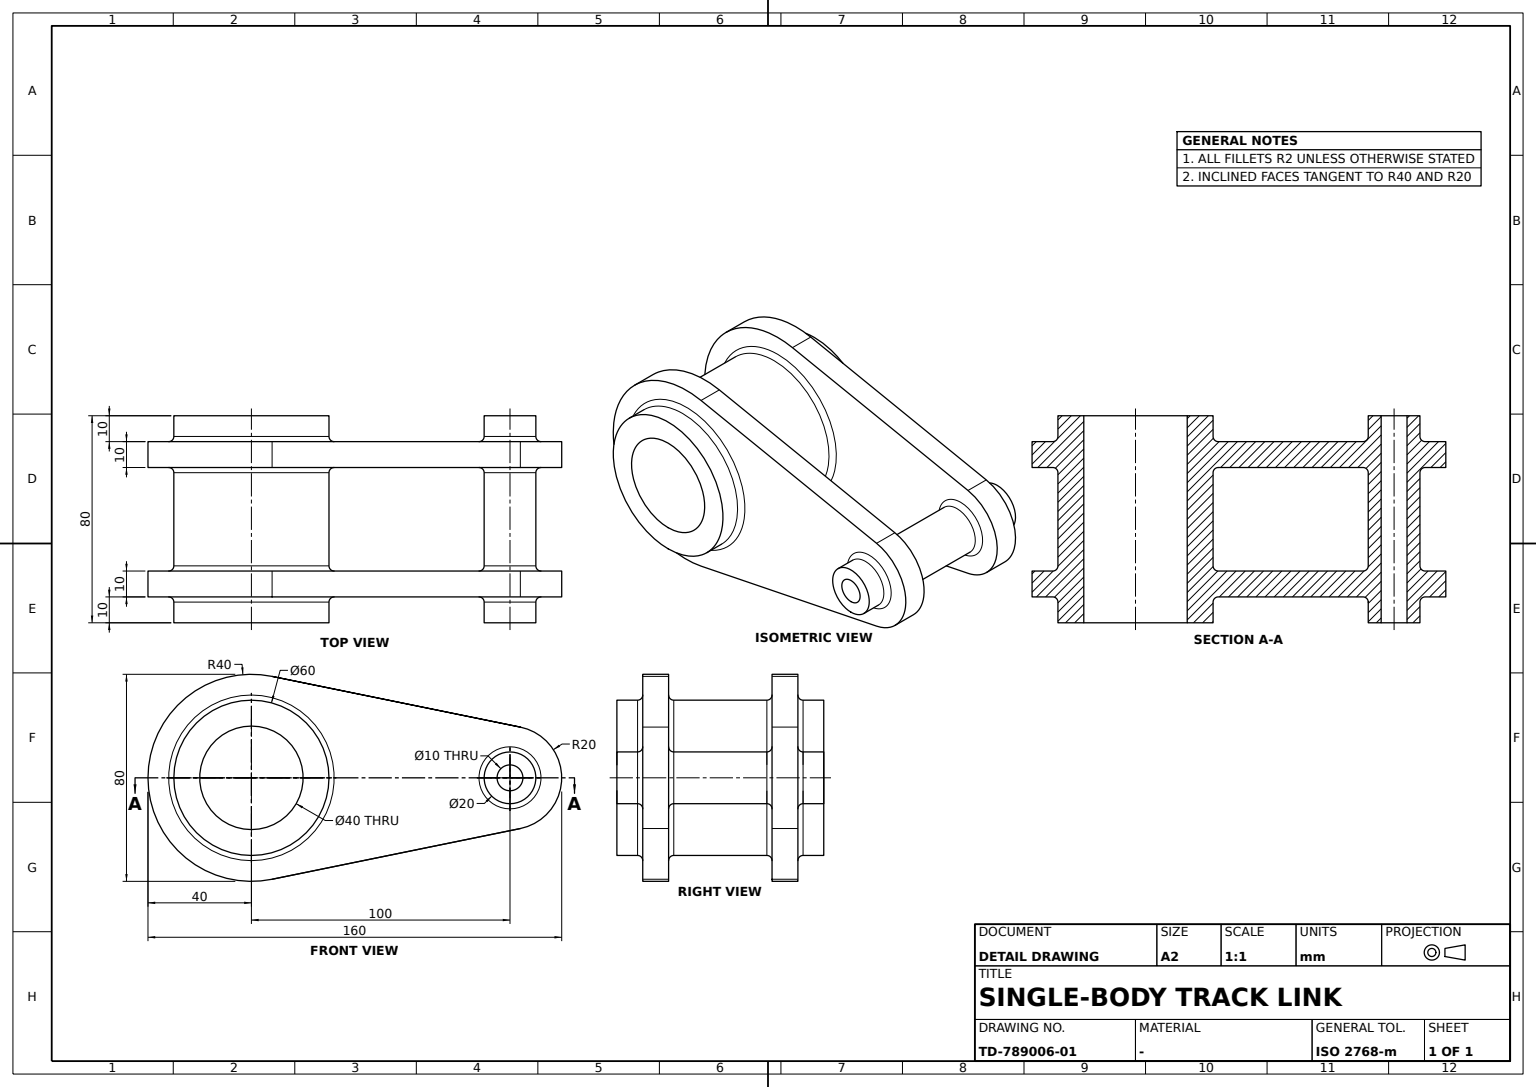
ISO-10303-21;
HEADER;
FILE_DESCRIPTION((''),'2;1');
FILE_NAME('','',(''),(''),'','','');
FILE_SCHEMA(('AUTOMOTIVE_DESIGN'));
ENDSEC;
DATA;
#1=APPLICATION_CONTEXT('');
#2=PRODUCT_CONTEXT('',#1,'mechanical');
#3=PRODUCT('','','',(#2));
#4=PRODUCT_DEFINITION_FORMATION('','',#3);
#5=PRODUCT_DEFINITION_CONTEXT('',#1,'design');
#6=PRODUCT_DEFINITION('','',#4,#5);
#7=PRODUCT_DEFINITION_SHAPE('','',#6);
#8=(LENGTH_UNIT()NAMED_UNIT(*)SI_UNIT(.MILLI.,.METRE.));
#9=(NAMED_UNIT(*)PLANE_ANGLE_UNIT()SI_UNIT($,.RADIAN.));
#10=(NAMED_UNIT(*)SI_UNIT($,.STERADIAN.)SOLID_ANGLE_UNIT());
#11=UNCERTAINTY_MEASURE_WITH_UNIT(LENGTH_MEASURE(0.005),#8,'distance_accuracy_value','');
#12=(GEOMETRIC_REPRESENTATION_CONTEXT(3)GLOBAL_UNCERTAINTY_ASSIGNED_CONTEXT((#11))GLOBAL_UNIT_ASSIGNED_CONTEXT((#8,#9,#10))REPRESENTATION_CONTEXT('',''));
#13=CARTESIAN_POINT('',(0.,103.999996,19.595919));
#14=VERTEX_POINT('',#13);
#15=CARTESIAN_POINT('',(10.,104.,19.595918));
#16=VERTEX_POINT('',#15);
#17=CARTESIAN_POINT('',(-45.,104.,19.595918));
#18=DIRECTION('',(-1.,0.,0.));
#19=VECTOR('',#18,1000.);
#20=LINE('',#17,#19);
#21=EDGE_CURVE('',#14,#16,#20,.F.);
#22=ORIENTED_EDGE('',*,*,#21,.F.);
#23=CARTESIAN_POINT('',(0.,8.,39.191836));
#24=VERTEX_POINT('',#23);
#25=DIRECTION('',(0.,0.979795897,-0.2));
#26=VECTOR('',#25,1000.);
#27=LINE('',#23,#26);
#28=EDGE_CURVE('',#24,#14,#27,.T.);
#29=ORIENTED_EDGE('',*,*,#28,.F.);
#30=CARTESIAN_POINT('',(10.,8.000004,39.191835));
#31=VERTEX_POINT('',#30);
#32=CARTESIAN_POINT('',(-45.,8.,39.191836));
#33=LINE('',#32,#19);
#34=EDGE_CURVE('',#24,#31,#33,.F.);
#35=ORIENTED_EDGE('',*,*,#34,.T.);
#36=CARTESIAN_POINT('',(10.,8.,39.191836));
#37=LINE('',#36,#26);
#38=EDGE_CURVE('',#31,#16,#37,.T.);
#39=ORIENTED_EDGE('',*,*,#38,.T.);
#40=EDGE_LOOP('',(#22,#29,#35,#39));
#41=FACE_BOUND('',#40,.T.);
#42=DIRECTION('',(0.,-0.2,-0.979795897));
#43=AXIS2_PLACEMENT_3D('',#23,#42,#25);
#44=PLANE('',#43);
#45=ADVANCED_FACE('',(#41),#44,.F.);
#46=ORIENTED_EDGE('',*,*,#34,.F.);
#47=CARTESIAN_POINT('',(0.,8.000004,-39.191835));
#48=VERTEX_POINT('',#47);
#49=CARTESIAN_POINT('',(0.,0.,0.));
#50=DIRECTION('',(1.,0.,0.));
#51=DIRECTION('',(0.,0.,-1.));
#52=AXIS2_PLACEMENT_3D('',#49,#50,#51);
#53=CIRCLE('',#52,40.);
#54=EDGE_CURVE('',#24,#48,#53,.T.);
#55=ORIENTED_EDGE('',*,*,#54,.T.);
#56=CARTESIAN_POINT('',(10.,8.,-39.191836));
#57=VERTEX_POINT('',#56);
#58=CARTESIAN_POINT('',(-45.,8.,-39.191836));
#59=LINE('',#58,#19);
#60=EDGE_CURVE('',#48,#57,#59,.F.);
#61=ORIENTED_EDGE('',*,*,#60,.T.);
#62=CARTESIAN_POINT('',(10.,0.,0.));
#63=AXIS2_PLACEMENT_3D('',#62,#50,#51);
#64=CIRCLE('',#63,40.);
#65=EDGE_CURVE('',#31,#57,#64,.T.);
#66=ORIENTED_EDGE('',*,*,#65,.F.);
#67=EDGE_LOOP('',(#46,#55,#61,#66));
#68=FACE_BOUND('',#67,.T.);
#69=CARTESIAN_POINT('',(-45.,0.,0.));
#70=DIRECTION('',(0.,-1.,0.));
#71=AXIS2_PLACEMENT_3D('',#69,#18,#70);
#72=CYLINDRICAL_SURFACE('',#71,40.);
#73=ADVANCED_FACE('',(#68),#72,.T.);
#74=CARTESIAN_POINT('',(-50.,104.,19.595918));
#75=VERTEX_POINT('',#74);
#76=CARTESIAN_POINT('',(-50.,104.,-19.595918));
#77=VERTEX_POINT('',#76);
#78=CARTESIAN_POINT('',(-50.,100.,0.));
#79=DIRECTION('',(0.,0.,1.));
#80=AXIS2_PLACEMENT_3D('',#78,#18,#79);
#81=CIRCLE('',#80,20.);
#82=EDGE_CURVE('',#75,#77,#81,.T.);
#83=ORIENTED_EDGE('',*,*,#82,.F.);
#84=CARTESIAN_POINT('',(-40.,104.,19.595918));
#85=VERTEX_POINT('',#84);
#86=EDGE_CURVE('',#85,#75,#20,.T.);
#87=ORIENTED_EDGE('',*,*,#86,.F.);
#88=CARTESIAN_POINT('',(-40.,104.,-19.595918));
#89=VERTEX_POINT('',#88);
#90=CARTESIAN_POINT('',(-40.,100.,0.));
#91=AXIS2_PLACEMENT_3D('',#90,#18,#79);
#92=CIRCLE('',#91,20.);
#93=EDGE_CURVE('',#85,#89,#92,.T.);
#94=ORIENTED_EDGE('',*,*,#93,.T.);
#95=CARTESIAN_POINT('',(-45.,104.,-19.595918));
#96=LINE('',#95,#19);
#97=EDGE_CURVE('',#89,#77,#96,.T.);
#98=ORIENTED_EDGE('',*,*,#97,.T.);
#99=EDGE_LOOP('',(#83,#87,#94,#98));
#100=FACE_BOUND('',#99,.T.);
#101=CARTESIAN_POINT('',(-45.,100.,0.));
#102=AXIS2_PLACEMENT_3D('',#101,#18,#70);
#103=CYLINDRICAL_SURFACE('',#102,20.);
#104=ADVANCED_FACE('',(#100),#103,.T.);
#105=CARTESIAN_POINT('',(20.,0.,-20.));
#106=VERTEX_POINT('',#105);
#107=CARTESIAN_POINT('',(20.,0.,0.));
#108=AXIS2_PLACEMENT_3D('',#107,#50,#51);
#109=CIRCLE('',#108,20.);
#110=EDGE_CURVE('',#106,#106,#109,.T.);
#111=ORIENTED_EDGE('',*,*,#110,.F.);
#112=EDGE_LOOP('',(#111));
#113=FACE_BOUND('',#112,.T.);
#114=CARTESIAN_POINT('',(20.,0.,-30.));
#115=VERTEX_POINT('',#114);
#116=CIRCLE('',#108,30.);
#117=EDGE_CURVE('',#115,#115,#116,.T.);
#118=ORIENTED_EDGE('',*,*,#117,.T.);
#119=EDGE_LOOP('',(#118));
#120=FACE_BOUND('',#119,.T.);
#121=DIRECTION('',(0.,1.,0.));
#122=AXIS2_PLACEMENT_3D('',#107,#50,#121);
#123=PLANE('',#122);
#124=ADVANCED_FACE('',(#113,#120),#123,.T.);
#125=CARTESIAN_POINT('',(-50.,100.,12.));
#126=VERTEX_POINT('',#125);
#127=CIRCLE('',#80,12.);
#128=EDGE_CURVE('',#126,#126,#127,.T.);
#129=ORIENTED_EDGE('',*,*,#128,.T.);
#130=EDGE_LOOP('',(#129));
#131=FACE_BOUND('',#130,.T.);
#132=CARTESIAN_POINT('',(-52.,100.,10.));
#133=VERTEX_POINT('',#132);
#134=CARTESIAN_POINT('',(-52.,100.,0.));
#135=AXIS2_PLACEMENT_3D('',#134,#18,#79);
#136=CIRCLE('',#135,10.);
#137=EDGE_CURVE('',#133,#133,#136,.T.);
#138=ORIENTED_EDGE('',*,*,#137,.F.);
#139=EDGE_LOOP('',(#138));
#140=FACE_BOUND('',#139,.T.);
#141=DIRECTION('',(0.,-0.707106781,-0.707106781));
#142=AXIS2_PLACEMENT_3D('',#134,#18,#141);
#143=TOROIDAL_SURFACE('',#142,12.,2.);
#144=ADVANCED_FACE('',(#131,#140),#143,.F.);
#145=CARTESIAN_POINT('',(0.,100.,-12.));
#146=VERTEX_POINT('',#145);
#147=CARTESIAN_POINT('',(0.,100.,0.));
#148=AXIS2_PLACEMENT_3D('',#147,#50,#51);
#149=CIRCLE('',#148,12.);
#150=EDGE_CURVE('',#146,#146,#149,.T.);
#151=ORIENTED_EDGE('',*,*,#150,.F.);
#152=EDGE_LOOP('',(#151));
#153=FACE_BOUND('',#152,.T.);
#154=CARTESIAN_POINT('',(-2.,100.,10.));
#155=VERTEX_POINT('',#154);
#156=CARTESIAN_POINT('',(-2.,100.,0.));
#157=AXIS2_PLACEMENT_3D('',#156,#18,#79);
#158=CIRCLE('',#157,10.);
#159=EDGE_CURVE('',#155,#155,#158,.F.);
#160=ORIENTED_EDGE('',*,*,#159,.T.);
#161=EDGE_LOOP('',(#160));
#162=FACE_BOUND('',#161,.T.);
#163=DIRECTION('',(0.,0.356808666,-0.934177486));
#164=AXIS2_PLACEMENT_3D('',#156,#50,#163);
#165=TOROIDAL_SURFACE('',#164,12.,2.);
#166=ADVANCED_FACE('',(#153,#162),#165,.F.);
#167=CARTESIAN_POINT('',(-60.,100.,5.));
#168=VERTEX_POINT('',#167);
#169=CARTESIAN_POINT('',(-60.,100.,0.));
#170=AXIS2_PLACEMENT_3D('',#169,#18,#79);
#171=CIRCLE('',#170,5.);
#172=EDGE_CURVE('',#168,#168,#171,.T.);
#173=ORIENTED_EDGE('',*,*,#172,.F.);
#174=EDGE_LOOP('',(#173));
#175=FACE_BOUND('',#174,.T.);
#176=CARTESIAN_POINT('',(-60.,100.,10.));
#177=VERTEX_POINT('',#176);
#178=CIRCLE('',#170,10.);
#179=EDGE_CURVE('',#177,#177,#178,.T.);
#180=ORIENTED_EDGE('',*,*,#179,.T.);
#181=EDGE_LOOP('',(#180));
#182=FACE_BOUND('',#181,.T.);
#183=CARTESIAN_POINT('',(-60.,0.,0.));
#184=AXIS2_PLACEMENT_3D('',#183,#18,#70);
#185=PLANE('',#184);
#186=ADVANCED_FACE('',(#175,#182),#185,.T.);
#187=CARTESIAN_POINT('',(10.,100.,-12.));
#188=VERTEX_POINT('',#187);
#189=CARTESIAN_POINT('',(10.,100.,0.));
#190=AXIS2_PLACEMENT_3D('',#189,#50,#51);
#191=CIRCLE('',#190,12.);
#192=EDGE_CURVE('',#188,#188,#191,.T.);
#193=ORIENTED_EDGE('',*,*,#192,.T.);
#194=EDGE_LOOP('',(#193));
#195=FACE_BOUND('',#194,.T.);
#196=CARTESIAN_POINT('',(12.,100.,10.));
#197=VERTEX_POINT('',#196);
#198=CARTESIAN_POINT('',(12.,100.,0.));
#199=AXIS2_PLACEMENT_3D('',#198,#18,#79);
#200=CIRCLE('',#199,10.);
#201=EDGE_CURVE('',#197,#197,#200,.F.);
#202=ORIENTED_EDGE('',*,*,#201,.F.);
#203=EDGE_LOOP('',(#202));
#204=FACE_BOUND('',#203,.T.);
#205=DIRECTION('',(0.,0.707106781,-0.707106781));
#206=AXIS2_PLACEMENT_3D('',#198,#50,#205);
#207=TOROIDAL_SURFACE('',#206,12.,2.);
#208=ADVANCED_FACE('',(#195,#204),#207,.F.);
#209=CARTESIAN_POINT('',(12.,0.,30.));
#210=VERTEX_POINT('',#209);
#211=CARTESIAN_POINT('',(12.,0.,0.));
#212=AXIS2_PLACEMENT_3D('',#211,#18,#79);
#213=CIRCLE('',#212,30.);
#214=EDGE_CURVE('',#210,#210,#213,.F.);
#215=ORIENTED_EDGE('',*,*,#214,.F.);
#216=EDGE_LOOP('',(#215));
#217=FACE_BOUND('',#216,.T.);
#218=CARTESIAN_POINT('',(10.,0.,-32.));
#219=VERTEX_POINT('',#218);
#220=CIRCLE('',#63,32.);
#221=EDGE_CURVE('',#219,#219,#220,.T.);
#222=ORIENTED_EDGE('',*,*,#221,.T.);
#223=EDGE_LOOP('',(#222));
#224=FACE_BOUND('',#223,.T.);
#225=DIRECTION('',(0.,0.677625322,-0.735407318));
#226=AXIS2_PLACEMENT_3D('',#211,#50,#225);
#227=TOROIDAL_SURFACE('',#226,32.,2.);
#228=ADVANCED_FACE('',(#217,#224),#227,.F.);
#229=CARTESIAN_POINT('',(-50.,8.,39.191836));
#230=VERTEX_POINT('',#229);
#231=LINE('',#229,#26);
#232=EDGE_CURVE('',#230,#75,#231,.T.);
#233=ORIENTED_EDGE('',*,*,#232,.F.);
#234=CARTESIAN_POINT('',(-40.,8.,39.191836));
#235=VERTEX_POINT('',#234);
#236=EDGE_CURVE('',#235,#230,#33,.T.);
#237=ORIENTED_EDGE('',*,*,#236,.F.);
#238=LINE('',#234,#26);
#239=EDGE_CURVE('',#235,#85,#238,.T.);
#240=ORIENTED_EDGE('',*,*,#239,.T.);
#241=ORIENTED_EDGE('',*,*,#86,.T.);
#242=EDGE_LOOP('',(#233,#237,#240,#241));
#243=FACE_BOUND('',#242,.T.);
#244=ADVANCED_FACE('',(#243),#44,.F.);
#245=ORIENTED_EDGE('',*,*,#150,.T.);
#246=EDGE_LOOP('',(#245));
#247=FACE_BOUND('',#246,.T.);
#248=ORIENTED_EDGE('',*,*,#54,.F.);
#249=ORIENTED_EDGE('',*,*,#28,.T.);
#250=CARTESIAN_POINT('',(0.,104.,-19.595918));
#251=VERTEX_POINT('',#250);
#252=CIRCLE('',#148,20.);
#253=EDGE_CURVE('',#251,#14,#252,.T.);
#254=ORIENTED_EDGE('',*,*,#253,.F.);
#255=CARTESIAN_POINT('',(0.,8.,-39.191836));
#256=DIRECTION('',(0.,0.979795897,0.2));
#257=VECTOR('',#256,1000.);
#258=LINE('',#255,#257);
#259=EDGE_CURVE('',#48,#251,#258,.T.);
#260=ORIENTED_EDGE('',*,*,#259,.F.);
#261=EDGE_LOOP('',(#248,#249,#254,#260));
#262=FACE_BOUND('',#261,.T.);
#263=CARTESIAN_POINT('',(0.,0.,-32.));
#264=VERTEX_POINT('',#263);
#265=CIRCLE('',#52,32.);
#266=EDGE_CURVE('',#264,#264,#265,.T.);
#267=ORIENTED_EDGE('',*,*,#266,.T.);
#268=EDGE_LOOP('',(#267));
#269=FACE_BOUND('',#268,.T.);
#270=AXIS2_PLACEMENT_3D('',#49,#50,#121);
#271=PLANE('',#270);
#272=ADVANCED_FACE('',(#247,#262,#269),#271,.F.);
#273=CARTESIAN_POINT('',(20.,100.,-5.));
#274=VERTEX_POINT('',#273);
#275=CARTESIAN_POINT('',(20.,100.,0.));
#276=AXIS2_PLACEMENT_3D('',#275,#50,#51);
#277=CIRCLE('',#276,5.);
#278=EDGE_CURVE('',#274,#274,#277,.T.);
#279=ORIENTED_EDGE('',*,*,#278,.T.);
#280=EDGE_LOOP('',(#279));
#281=FACE_BOUND('',#280,.T.);
#282=ORIENTED_EDGE('',*,*,#172,.T.);
#283=EDGE_LOOP('',(#282));
#284=FACE_BOUND('',#283,.T.);
#285=CARTESIAN_POINT('',(-20.,100.,0.));
#286=AXIS2_PLACEMENT_3D('',#285,#18,#70);
#287=CYLINDRICAL_SURFACE('',#286,5.);
#288=ADVANCED_FACE('',(#281,#284),#287,.F.);
#289=ORIENTED_EDGE('',*,*,#278,.F.);
#290=EDGE_LOOP('',(#289));
#291=FACE_BOUND('',#290,.T.);
#292=CARTESIAN_POINT('',(20.,100.,-10.));
#293=VERTEX_POINT('',#292);
#294=CIRCLE('',#276,10.);
#295=EDGE_CURVE('',#293,#293,#294,.T.);
#296=ORIENTED_EDGE('',*,*,#295,.T.);
#297=EDGE_LOOP('',(#296));
#298=FACE_BOUND('',#297,.T.);
#299=ADVANCED_FACE('',(#291,#298),#123,.T.);
#300=ORIENTED_EDGE('',*,*,#179,.F.);
#301=EDGE_LOOP('',(#300));
#302=FACE_BOUND('',#301,.T.);
#303=ORIENTED_EDGE('',*,*,#137,.T.);
#304=EDGE_LOOP('',(#303));
#305=FACE_BOUND('',#304,.T.);
#306=CYLINDRICAL_SURFACE('',#286,10.);
#307=ADVANCED_FACE('',(#302,#305),#306,.T.);
#308=ORIENTED_EDGE('',*,*,#239,.F.);
#309=CARTESIAN_POINT('',(-40.,8.,-39.191836));
#310=VERTEX_POINT('',#309);
#311=CARTESIAN_POINT('',(-40.,0.,0.));
#312=AXIS2_PLACEMENT_3D('',#311,#18,#79);
#313=CIRCLE('',#312,40.);
#314=EDGE_CURVE('',#310,#235,#313,.T.);
#315=ORIENTED_EDGE('',*,*,#314,.F.);
#316=LINE('',#309,#257);
#317=EDGE_CURVE('',#310,#89,#316,.T.);
#318=ORIENTED_EDGE('',*,*,#317,.T.);
#319=ORIENTED_EDGE('',*,*,#93,.F.);
#320=EDGE_LOOP('',(#308,#315,#318,#319));
#321=FACE_BOUND('',#320,.T.);
#322=CARTESIAN_POINT('',(-40.,100.,12.));
#323=VERTEX_POINT('',#322);
#324=CIRCLE('',#91,12.);
#325=EDGE_CURVE('',#323,#323,#324,.T.);
#326=ORIENTED_EDGE('',*,*,#325,.T.);
#327=EDGE_LOOP('',(#326));
#328=FACE_BOUND('',#327,.T.);
#329=CARTESIAN_POINT('',(-40.,0.,32.));
#330=VERTEX_POINT('',#329);
#331=CIRCLE('',#312,32.);
#332=EDGE_CURVE('',#330,#330,#331,.T.);
#333=ORIENTED_EDGE('',*,*,#332,.T.);
#334=EDGE_LOOP('',(#333));
#335=FACE_BOUND('',#334,.T.);
#336=AXIS2_PLACEMENT_3D('',#311,#18,#70);
#337=PLANE('',#336);
#338=ADVANCED_FACE('',(#321,#328,#335),#337,.F.);
#339=ORIENTED_EDGE('',*,*,#253,.T.);
#340=ORIENTED_EDGE('',*,*,#21,.T.);
#341=CARTESIAN_POINT('',(10.,103.999996,-19.595919));
#342=VERTEX_POINT('',#341);
#343=CIRCLE('',#190,20.);
#344=EDGE_CURVE('',#342,#16,#343,.T.);
#345=ORIENTED_EDGE('',*,*,#344,.F.);
#346=EDGE_CURVE('',#251,#342,#96,.F.);
#347=ORIENTED_EDGE('',*,*,#346,.F.);
#348=EDGE_LOOP('',(#339,#340,#345,#347));
#349=FACE_BOUND('',#348,.T.);
#350=ADVANCED_FACE('',(#349),#103,.T.);
#351=ORIENTED_EDGE('',*,*,#159,.F.);
#352=EDGE_LOOP('',(#351));
#353=FACE_BOUND('',#352,.T.);
#354=CARTESIAN_POINT('',(-38.,100.,10.));
#355=VERTEX_POINT('',#354);
#356=CARTESIAN_POINT('',(-38.,100.,0.));
#357=AXIS2_PLACEMENT_3D('',#356,#18,#79);
#358=CIRCLE('',#357,10.);
#359=EDGE_CURVE('',#355,#355,#358,.T.);
#360=ORIENTED_EDGE('',*,*,#359,.F.);
#361=EDGE_LOOP('',(#360));
#362=FACE_BOUND('',#361,.T.);
#363=ADVANCED_FACE('',(#353,#362),#306,.T.);
#364=CARTESIAN_POINT('',(-60.,0.,30.));
#365=VERTEX_POINT('',#364);
#366=AXIS2_PLACEMENT_3D('',#183,#18,#79);
#367=CIRCLE('',#366,30.);
#368=EDGE_CURVE('',#365,#365,#367,.T.);
#369=ORIENTED_EDGE('',*,*,#368,.T.);
#370=EDGE_LOOP('',(#369));
#371=FACE_BOUND('',#370,.T.);
#372=CARTESIAN_POINT('',(-60.,0.,20.));
#373=VERTEX_POINT('',#372);
#374=CIRCLE('',#366,20.);
#375=EDGE_CURVE('',#373,#373,#374,.T.);
#376=ORIENTED_EDGE('',*,*,#375,.F.);
#377=EDGE_LOOP('',(#376));
#378=FACE_BOUND('',#377,.T.);
#379=ADVANCED_FACE('',(#371,#378),#185,.T.);
#380=CARTESIAN_POINT('',(-50.,8.,-39.191836));
#381=VERTEX_POINT('',#380);
#382=LINE('',#380,#257);
#383=EDGE_CURVE('',#381,#77,#382,.T.);
#384=ORIENTED_EDGE('',*,*,#383,.T.);
#385=ORIENTED_EDGE('',*,*,#97,.F.);
#386=ORIENTED_EDGE('',*,*,#317,.F.);
#387=EDGE_CURVE('',#310,#381,#59,.T.);
#388=ORIENTED_EDGE('',*,*,#387,.T.);
#389=EDGE_LOOP('',(#384,#385,#386,#388));
#390=FACE_BOUND('',#389,.T.);
#391=DIRECTION('',(0.,0.2,-0.979795897));
#392=AXIS2_PLACEMENT_3D('',#255,#391,#256);
#393=PLANE('',#392);
#394=ADVANCED_FACE('',(#390),#393,.T.);
#395=ORIENTED_EDGE('',*,*,#214,.T.);
#396=EDGE_LOOP('',(#395));
#397=FACE_BOUND('',#396,.T.);
#398=ORIENTED_EDGE('',*,*,#117,.F.);
#399=EDGE_LOOP('',(#398));
#400=FACE_BOUND('',#399,.T.);
#401=CARTESIAN_POINT('',(-20.,0.,0.));
#402=AXIS2_PLACEMENT_3D('',#401,#18,#70);
#403=CYLINDRICAL_SURFACE('',#402,30.);
#404=ADVANCED_FACE('',(#397,#400),#403,.T.);
#405=ORIENTED_EDGE('',*,*,#375,.T.);
#406=EDGE_LOOP('',(#405));
#407=FACE_BOUND('',#406,.T.);
#408=ORIENTED_EDGE('',*,*,#110,.T.);
#409=EDGE_LOOP('',(#408));
#410=FACE_BOUND('',#409,.T.);
#411=CYLINDRICAL_SURFACE('',#402,20.);
#412=ADVANCED_FACE('',(#407,#410),#411,.F.);
#413=ORIENTED_EDGE('',*,*,#314,.T.);
#414=ORIENTED_EDGE('',*,*,#236,.T.);
#415=CARTESIAN_POINT('',(-50.,0.,0.));
#416=AXIS2_PLACEMENT_3D('',#415,#18,#79);
#417=CIRCLE('',#416,40.);
#418=EDGE_CURVE('',#381,#230,#417,.T.);
#419=ORIENTED_EDGE('',*,*,#418,.F.);
#420=ORIENTED_EDGE('',*,*,#387,.F.);
#421=EDGE_LOOP('',(#413,#414,#419,#420));
#422=FACE_BOUND('',#421,.T.);
#423=ADVANCED_FACE('',(#422),#72,.T.);
#424=ORIENTED_EDGE('',*,*,#332,.F.);
#425=EDGE_LOOP('',(#424));
#426=FACE_BOUND('',#425,.T.);
#427=CARTESIAN_POINT('',(-38.,0.,30.));
#428=VERTEX_POINT('',#427);
#429=CARTESIAN_POINT('',(-38.,0.,0.));
#430=AXIS2_PLACEMENT_3D('',#429,#18,#79);
#431=CIRCLE('',#430,30.);
#432=EDGE_CURVE('',#428,#428,#431,.T.);
#433=ORIENTED_EDGE('',*,*,#432,.T.);
#434=EDGE_LOOP('',(#433));
#435=FACE_BOUND('',#434,.T.);
#436=DIRECTION('',(0.,-0.646991665,-0.762497072));
#437=AXIS2_PLACEMENT_3D('',#429,#18,#436);
#438=TOROIDAL_SURFACE('',#437,32.,2.);
#439=ADVANCED_FACE('',(#426,#435),#438,.F.);
#440=ORIENTED_EDGE('',*,*,#325,.F.);
#441=EDGE_LOOP('',(#440));
#442=FACE_BOUND('',#441,.T.);
#443=ORIENTED_EDGE('',*,*,#359,.T.);
#444=EDGE_LOOP('',(#443));
#445=FACE_BOUND('',#444,.T.);
#446=DIRECTION('',(0.,-0.658267857,-0.752783786));
#447=AXIS2_PLACEMENT_3D('',#356,#18,#446);
#448=TOROIDAL_SURFACE('',#447,12.,2.);
#449=ADVANCED_FACE('',(#442,#445),#448,.F.);
#450=CARTESIAN_POINT('',(-2.,0.,30.));
#451=VERTEX_POINT('',#450);
#452=CARTESIAN_POINT('',(-2.,0.,0.));
#453=AXIS2_PLACEMENT_3D('',#452,#18,#79);
#454=CIRCLE('',#453,30.);
#455=EDGE_CURVE('',#451,#451,#454,.F.);
#456=ORIENTED_EDGE('',*,*,#455,.T.);
#457=EDGE_LOOP('',(#456));
#458=FACE_BOUND('',#457,.T.);
#459=ORIENTED_EDGE('',*,*,#266,.F.);
#460=EDGE_LOOP('',(#459));
#461=FACE_BOUND('',#460,.T.);
#462=DIRECTION('',(0.,0.486033264,-0.87394031));
#463=AXIS2_PLACEMENT_3D('',#452,#50,#462);
#464=TOROIDAL_SURFACE('',#463,32.,2.);
#465=ADVANCED_FACE('',(#458,#461),#464,.F.);
#466=ORIENTED_EDGE('',*,*,#295,.F.);
#467=EDGE_LOOP('',(#466));
#468=FACE_BOUND('',#467,.T.);
#469=ORIENTED_EDGE('',*,*,#201,.T.);
#470=EDGE_LOOP('',(#469));
#471=FACE_BOUND('',#470,.T.);
#472=ADVANCED_FACE('',(#468,#471),#306,.T.);
#473=ORIENTED_EDGE('',*,*,#232,.T.);
#474=ORIENTED_EDGE('',*,*,#82,.T.);
#475=ORIENTED_EDGE('',*,*,#383,.F.);
#476=ORIENTED_EDGE('',*,*,#418,.T.);
#477=EDGE_LOOP('',(#473,#474,#475,#476));
#478=FACE_BOUND('',#477,.T.);
#479=ORIENTED_EDGE('',*,*,#128,.F.);
#480=EDGE_LOOP('',(#479));
#481=FACE_BOUND('',#480,.T.);
#482=CARTESIAN_POINT('',(-50.,0.,32.));
#483=VERTEX_POINT('',#482);
#484=CIRCLE('',#416,32.);
#485=EDGE_CURVE('',#483,#483,#484,.T.);
#486=ORIENTED_EDGE('',*,*,#485,.F.);
#487=EDGE_LOOP('',(#486));
#488=FACE_BOUND('',#487,.T.);
#489=AXIS2_PLACEMENT_3D('',#415,#18,#70);
#490=PLANE('',#489);
#491=ADVANCED_FACE('',(#478,#481,#488),#490,.T.);
#492=ORIENTED_EDGE('',*,*,#192,.F.);
#493=EDGE_LOOP('',(#492));
#494=FACE_BOUND('',#493,.T.);
#495=ORIENTED_EDGE('',*,*,#38,.F.);
#496=ORIENTED_EDGE('',*,*,#65,.T.);
#497=LINE('',#56,#257);
#498=EDGE_CURVE('',#57,#342,#497,.T.);
#499=ORIENTED_EDGE('',*,*,#498,.T.);
#500=ORIENTED_EDGE('',*,*,#344,.T.);
#501=EDGE_LOOP('',(#495,#496,#499,#500));
#502=FACE_BOUND('',#501,.T.);
#503=ORIENTED_EDGE('',*,*,#221,.F.);
#504=EDGE_LOOP('',(#503));
#505=FACE_BOUND('',#504,.T.);
#506=AXIS2_PLACEMENT_3D('',#62,#50,#121);
#507=PLANE('',#506);
#508=ADVANCED_FACE('',(#494,#502,#505),#507,.T.);
#509=ORIENTED_EDGE('',*,*,#432,.F.);
#510=EDGE_LOOP('',(#509));
#511=FACE_BOUND('',#510,.T.);
#512=ORIENTED_EDGE('',*,*,#455,.F.);
#513=EDGE_LOOP('',(#512));
#514=FACE_BOUND('',#513,.T.);
#515=ADVANCED_FACE('',(#511,#514),#403,.T.);
#516=CARTESIAN_POINT('',(-52.,0.,30.));
#517=VERTEX_POINT('',#516);
#518=CARTESIAN_POINT('',(-52.,0.,0.));
#519=AXIS2_PLACEMENT_3D('',#518,#18,#79);
#520=CIRCLE('',#519,30.);
#521=EDGE_CURVE('',#517,#517,#520,.T.);
#522=ORIENTED_EDGE('',*,*,#521,.F.);
#523=EDGE_LOOP('',(#522));
#524=FACE_BOUND('',#523,.T.);
#525=ORIENTED_EDGE('',*,*,#485,.T.);
#526=EDGE_LOOP('',(#525));
#527=FACE_BOUND('',#526,.T.);
#528=DIRECTION('',(0.,-0.677625322,-0.735407318));
#529=AXIS2_PLACEMENT_3D('',#518,#18,#528);
#530=TOROIDAL_SURFACE('',#529,32.,2.);
#531=ADVANCED_FACE('',(#524,#527),#530,.F.);
#532=ORIENTED_EDGE('',*,*,#259,.T.);
#533=ORIENTED_EDGE('',*,*,#346,.T.);
#534=ORIENTED_EDGE('',*,*,#498,.F.);
#535=ORIENTED_EDGE('',*,*,#60,.F.);
#536=EDGE_LOOP('',(#532,#533,#534,#535));
#537=FACE_BOUND('',#536,.T.);
#538=ADVANCED_FACE('',(#537),#393,.T.);
#539=ORIENTED_EDGE('',*,*,#368,.F.);
#540=EDGE_LOOP('',(#539));
#541=FACE_BOUND('',#540,.T.);
#542=ORIENTED_EDGE('',*,*,#521,.T.);
#543=EDGE_LOOP('',(#542));
#544=FACE_BOUND('',#543,.T.);
#545=ADVANCED_FACE('',(#541,#544),#403,.T.);
#546=CLOSED_SHELL('',(#45,#73,#104,#124,#144,#166,#186,#208,#228,#244,#272,#288,#299,#307,#338,#350,#363,#379,#394,#404,#412,#423,#439,#449,#465,#472,#491,#508,#515,#531,#538,#545));
#547=MANIFOLD_SOLID_BREP('',#546);
#548=ADVANCED_BREP_SHAPE_REPRESENTATION('',(#547),#12);
#549=SHAPE_DEFINITION_REPRESENTATION(#7,#548);
ENDSEC;
END-ISO-10303-21;
